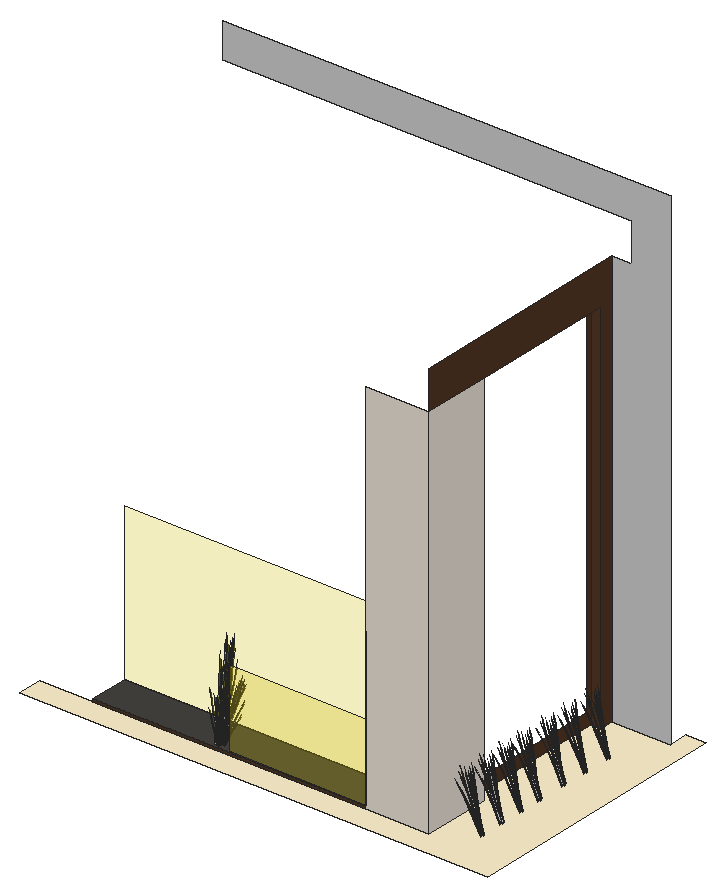
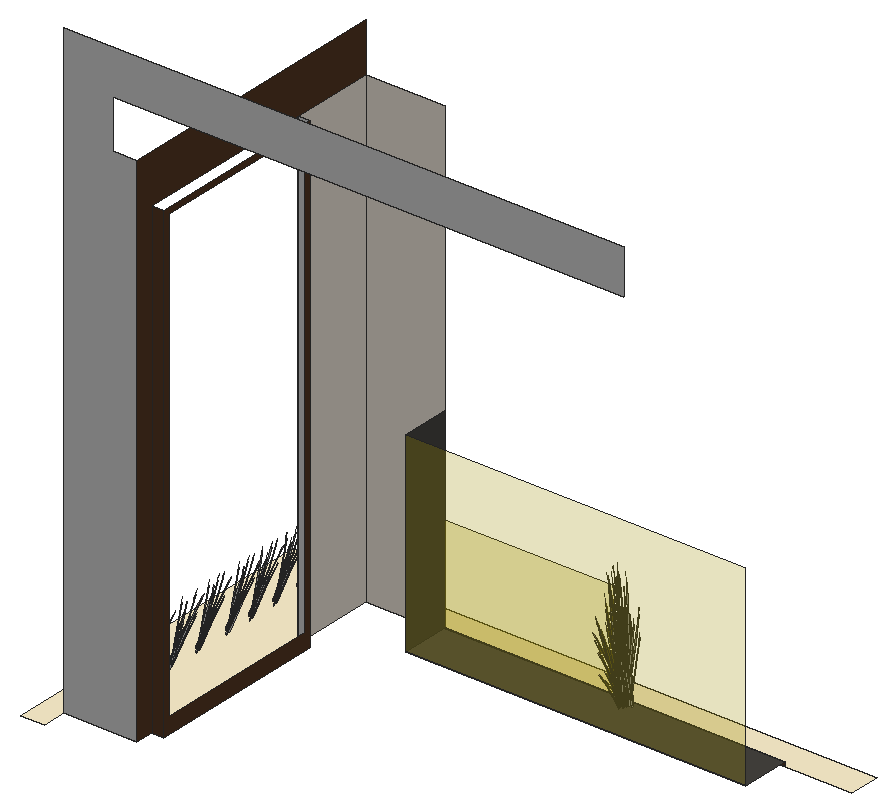
# SketchUp Ruby script. Lengths in inches.
U = 1.inch
M = Sketchup.active_model
def pt(a) = Geom::Point3d.new(a.map { |v| v * U })
def face(e, loops, mat)
  f = e.add_face(loops[0].map { |a| pt(a) })
  loops[1..].each { |l| e.add_face(l.map { |a| pt(a) }).erase! }
  f.material = f.back_material = mat if mat
  f
end
# faces: each face lists its corners as indices into pts; further lists are holes
def faces(e, pts, list, mat = nil) = list.each { |f| face(e, (f[0].is_a?(Array) ? f : [f]).map { |l| l.map { |i| pts[i] } }, mat) }
# xy, xz, yz: faces in a plane at the given z, y or x. An outline is a flat list of corners, or four numbers for a rectangle; further outlines are holes
def ring(l) = l.size == 4 ? [[l[0], l[1]], [l[2], l[1]], [l[2], l[3]], [l[0], l[3]]] : l.each_slice(2).to_a
def flat(e, list, mat, &to3) = list.each { |f| face(e, (f[0].is_a?(Array) ? f : [f]).map { |l| ring(l).map { |u, v| to3.(u, v) } }, mat) }
def xy(e, z, list, mat = nil) = flat(e, list, mat) { |x, y| [x, y, z] }
def xz(e, y, list, mat = nil) = flat(e, list, mat) { |x, z| [x, y, z] }
def yz(e, x, list, mat = nil) = flat(e, list, mat) { |y, z| [x, y, z] }
def lines(e, pts, list) = list.each { |a, b| e.add_line(pt(pts[a]), pt(pts[b])) }
# prism: a flat outline (further loops are holes) pulled along v
def prism(e, loops, v, mat = nil)
  f = face(e, loops, mat); d = Geom::Vector3d.new(v.map { |x| x * U })
  f.pushpull(f.normal.samedirection?(d) ? d.length : -d.length)
end
def box(e, o, s, mat = nil) = prism(e, [[o, [o[0] + s[0], o[1], o[2]], [o[0] + s[0], o[1] + s[1], o[2]], [o[0], o[1] + s[1], o[2]]]], [0, 0, s[2]], mat)
def at(x, y, z, deg = 0) = Geom::Transformation.translation(pt([x, y, z])) * Geom::Transformation.rotation(ORIGIN, Z_AXIS, deg.degrees)
def axes(o, x, y, z) = Geom::Transformation.new([*x, 0, *y, 0, *z, 0, *pt(o).to_a, 1])
def part(name) = M.definitions.add(name)
# library, detail: a bought-in or finely detailed component or shape, given as its bounding box
def library(name, o, s) = part(name).tap { |d| box(d.entities, o, s) }
def detail(e, o, s) = box(e.add_group.entities, o, s)
def put(e, d, t, mat = nil) = e.add_instance(d, t).tap { |i| i.material = mat if mat }
def group(e, t, mat = nil) = e.add_group.tap { |g| g.transformation = t; g.material = mat if mat }.entities
root = M.entities
M.materials.add("D01_Frost_White").color = [255, 242, 206]
M.materials.add("Glass_Basic_01").color = [255, 228, 0]
M.materials["Glass_Basic_01"].alpha = 0.25
M.materials.add("LightPink_Translucent").color = [144, 107, 117]
M.materials["LightPink_Translucent"].alpha = 0.75
M.materials.add("Marble_01_1K").color = [230, 221, 211]
M.materials.add("Wood_Planks_01_1K").color = [69, 67, 63]
M.materials.add("Wood_Veneer_15_1K").color = [81, 54, 35]
M.materials.add("[_0053_Ivory_]").color = [200, 200, 200]
c1 = part("blade")
p = [[2.15,0.21,22],[0,0.17,0],[0.09,0.45,0],[2.18,0.31,22],[2.29,0.31,22],[0.38,0.45,0],
  [2.48,0.24,33],[2.49,0.24,33],[2.48,0.22,33]]
faces(c1.entities,p,[[0,1,2,3],[4,5,2,3],[6,3,4,7],[8,0,3,6]])
c2 = part("seeds")
p = [[0.3,-0.1,1.38],[-0.01,-0.03,1.59],[-0.01,-0.03,0.03],[0.14,-0.07,-0.07],[0.29,-0.03,3],[0.15,0.01,3.11]]
faces(c2.entities,p,[[0,1,2,3],[1,0,4,5]],"LightPink_Translucent")
c3 = part("blade with seeds")
put(c3.entities,c1,at(0,0,0))
put(c3.entities,c2,axes([2.4,0.25,30.99],[1.5799,-0.05474,1.17369],[-0.12525,1.92788,0.29478],[-0.07173,-0.02425,1.56792]))
xy(root,127,[[377.51,83.15,665.51,83.15,665.51,251.15,653.51,251.15,653.51,239.15,617.51,239.15,617.51,230.15,611.51,230.15,611.51,140.15,617.51,140.15,617.51,98.15,377.51,98.15]],"D01_Frost_White")
xy(root,129,[[410.51,98.15,578.51,122.15]],"Wood_Planks_01_1K")
xz(root,98.15,[[494.51,129,578.51,177]],"Glass_Basic_01")
xz(root,98.15,[[578.51,127,617.51,360]],"Marble_01_1K")
xz(root,98.15,[[410.51,127,578.51,129]],"Wood_Veneer_15_1K")
xz(root,122.15,[[410.51,129,578.51,225]],"Glass_Basic_01")
xz(root,140.15,[[611.51,127,617.51,360]],"[_0053_Ivory_]")
xz(root,230.15,[[611.51,127,617.51,360]],"Wood_Veneer_15_1K")
xz(root,239.15,[[617.51,127,653.51,127,653.51,430,377.51,430,377.51,408,629.51,408,629.51,384,617.51,384]],"[_0053_Ivory_]")
yz(root,578.51,[[98.15,129,122.15,225]],"Wood_Planks_01_1K")
yz(root,611.51,[[[140.15,127,230.15,360],[143.15,135,227.15,357]]],"Wood_Veneer_15_1K")
yz(root,617.51,[[98.15,127,140.15,360]],"Marble_01_1K")
yz(root,617.51,[[230.15,127,239.15,127,239.15,384,98.15,384,98.15,360,230.15,360]],"Wood_Veneer_15_1K")
put(root,c3,axes([484.17,100.16,128.68],[0.56663,0.1556,-0.30978],[-0.14267,0.54795,0.30978],[0.11423,-0.06319,1.38974]),"[_0053_Ivory_]")
put(root,c3,axes([485.75,99.5,129.24],[-0.17264,0.12729,1.43002],[-0.51703,-0.22279,-0.30754],[0.09584,-0.27707,0.61141]),"[_0053_Ivory_]")
put(root,c3,axes([487.11,102.46,129.13],[0,-0.62885,0.49651],[0.67951,0,0],[0,0.14322,1.57504]),"[_0053_Ivory_]")
put(root,c3,axes([487.4,103.04,128.67],[0,0.62885,-0.49651],[-0.67951,0,0],[0,0.14322,1.57504]),"[_0053_Ivory_]")
put(root,c3,axes([484.04,99.91,128.67],[0.56842,-0.31443,-0.49651],[0.33976,0.56381,0],[0.12946,-0.07161,1.57504]),"[_0053_Ivory_]")
put(root,c3,axes([484.77,103.74,130.53],[-0.13883,-0.2019,1.71376],[0.64153,-0.16998,0.13857],[0.14499,0.31697,0.73262]),"[_0053_Ivory_]")
put(root,c3,axes([485.18,101.47,129.27],[0.11717,-0.56122,0.1448],[0.57245,0.09742,-0.41347],[0.10418,0.05763,1.26744]),"[_0053_Ivory_]")
put(root,c3,axes([485.99,100.5,129.13],[-0.56842,-0.31443,0.49651],[0.33976,-0.56381,0],[0.12946,0.07161,1.57504]),"[_0053_Ivory_]")
put(root,c3,axes([486.17,100.44,131.63],[0.0158,-0.58168,-0.71045],[0.66548,0.03907,0.08574],[0.07023,-0.24643,1.00501]),"[_0053_Ivory_]")
put(root,c3,axes([485.5,103.78,128.84],[0.63764,-0.21337,-0.19198],[0.22406,0.61462,0.00008],[0.07038,-0.02358,1.73897]),"[_0053_Ivory_]")
put(root,c3,axes([485.51,101.95,128.86],[0.36485,0.52782,-0.44739],[-0.55265,0.37168,0.21531],[0.11807,0.06531,1.43643]),"[_0053_Ivory_]")
put(root,c3,axes([486.44,100.09,131.18],[0.41095,-0.33109,-0.35414],[0.38901,0.37805,0.4572],[0.05919,-0.19208,0.87481]),"[_0053_Ivory_]")
put(root,c3,axes([486.54,104.35,129.42],[-0.34197,-0.18082,1.1486],[0.44156,-0.18372,0.84392],[0.1191,0.15563,0.25299]),"[_0053_Ivory_]")
put(root,c3,axes([485.32,104.15,129.24],[0.01072,-0.20846,1.43002],[0.51218,-0.23285,-0.30754],[0.15811,0.2495,0.61141]),"[_0053_Ivory_]")
put(root,c3,axes([484.71,101.2,128.71],[0.40909,-0.47266,-0.62353],[0.50819,0.4286,-0.16365],[0.16393,-0.11791,1.37633]),"[_0053_Ivory_]")
put(root,c3,axes([486.51,100.78,128.68],[0.14267,0.54795,-0.30978],[-0.56663,0.1556,0.30978],[0.11423,0.06319,1.38974]),"[_0053_Ivory_]")
put(root,c3,axes([487.57,102.57,129.03],[0.75945,0,0],[0,0.70283,-0.51607],[0,0.16007,1.63711]),"[_0053_Ivory_]")
put(root,c3,axes([485.12,101.66,129.32],[0.61322,-0.4175,-0.29095],[0.40778,0.58992,-0.50002],[0.1513,0.05991,1.59708]),"[_0053_Ivory_]")
put(root,c3,axes([486.59,105.17,129.32],[-0.38947,-0.01972,1.0506],[0.25721,-0.41888,0.58006],[0.15386,0.14882,0.8241]),"[_0053_Ivory_]")
put(root,c3,axes([485.42,100.15,130.53],[-0.11309,0.21615,1.71376],[-0.47441,-0.44731,0.13857],[0.21402,-0.27879,0.73262]),"[_0053_Ivory_]")
put(root,c3,axes([483.57,101.28,128.25],[-0.59782,0.25177,1.28929],[-0.19028,-0.72239,0.50096],[0.36709,0.01202,1.46642]),"[_0053_Ivory_]")
put(root,c3,axes([485.77,104.6,131.33],[0.59932,-0.14948,-0.51099],[0.10484,0.56611,-0.3958],[0.16097,0.16223,0.97773]),"[_0053_Ivory_]")
put(root,c3,axes([486.32,100.17,129.03],[0.37973,-0.63014,0],[0.6353,0.35142,-0.51607],[0.14469,0.08004,1.63711]),"[_0053_Ivory_]")
put(root,c3,axes([486.95,99.89,128.15],[-0.0909,-0.04954,1.76342],[-0.2335,-0.55347,-0.26939],[0.15752,-0.1502,0.30037]),"[_0053_Ivory_]")
put(root,c3,axes([486.66,100.55,128.67],[0.56842,0.31443,-0.49651],[-0.33976,0.56381,0],[0.12946,0.07161,1.57504]),"[_0053_Ivory_]")
put(root,c3,axes([486.64,105.02,128.15],[0.04425,-0.09079,1.76342],[0.55709,-0.26738,-0.26939],[0.16889,0.13839,0.30037]),"[_0053_Ivory_]")
put(root,c3,axes([486.94,101.22,131.33],[-0.15602,-0.5742,-0.51099],[0.59087,-0.10045,-0.3958],[0.16933,-0.15423,0.97773]),"[_0053_Ivory_]")
put(root,c3,axes([487.97,104.18,130.58],[-0.11624,-0.52862,-0.03492],[0.54943,-0.12153,-0.15832],[0.11473,0.03351,0.52218]),"[_0053_Ivory_]")
put(root,c3,axes([485.84,101.75,128.71],[0.63179,0.1031,-0.62353],[-0.13332,0.63596,-0.16365],[0.18854,0.07706,1.37633]),"[_0053_Ivory_]")
put(root,c3,axes([488.53,102.125,128.91],[-0.37654,-0.40212,-0.06488],[0.4124,-0.36845,-0.29416],[0.11685,-0.02594,0.97024]),"[_0053_Ivory_]")
put(root,c3,axes([487.66,100.08,129.42],[-0.2023,0.32011,1.1486],[-0.17388,-0.43009,0.84392],[0.16708,-0.10777,0.25299]),"[_0053_Ivory_]")
put(root,c3,axes([485.7,103.11,130.53],[-0.2256,-0.10835,1.71376],[0.46687,-0.45453,0.13857],[0.29098,0.20505,0.73262]),"[_0053_Ivory_]")
put(root,c3,axes([487.37,101.28,131.18],[0.52868,-0.08987,-0.35414],[0.1396,0.51376,0.4572],[0.1515,-0.13799,0.87481]),"[_0053_Ivory_]")
put(root,c3,axes([486.95,101.45,131.63],[0.31725,-0.49618,-0.71045],[0.55593,0.35263,0.08574],[0.18942,-0.17977,1.00501]),"[_0053_Ivory_]")
put(root,c3,axes([486.95,104.12,131.18],[0.34557,0.39372,-0.35414],[-0.39459,0.37271,0.4572],[0.20048,0.05671,0.87481]),"[_0053_Ivory_]")
put(root,c3,axes([487.21,102.5,131.33],[0.16454,-0.57202,-0.51099],[0.56413,0.19607,-0.3958],[0.22713,-0.05245,0.97773]),"[_0053_Ivory_]")
put(root,c3,axes([488.625,102.86,129.42],[-0.37526,0.10382,1.1486],[0.17664,-0.42906,0.84392],[0.19907,0.02936,0.25299]),"[_0053_Ivory_]")
put(root,c3,axes([487.41,101,129.24],[-0.21697,-0.01863,1.43002],[-0.22228,-0.49966,-0.30754],[0.26655,-0.14135,0.61141]),"[_0053_Ivory_]")
put(root,c3,axes([487.56,102.76,131.18],[0.50475,0.17543,-0.35414],[-0.14722,0.5118,0.4572],[0.20322,-0.04693,0.87481]),"[_0053_Ivory_]")
put(root,c3,axes([486.58,103.86,131.63],[0.60713,0.01514,-0.71045],[-0.04078,0.63759,0.08574],[0.25721,0.06729,1.00501]),"[_0053_Ivory_]")
put(root,c3,axes([487.8125,102.66,128.64],[-0.39118,0.07547,1.41583],[-0.06226,-0.6007,0.08104],[0.27398,-0.09092,0.80566]),"[_0053_Ivory_]")
put(root,c3,axes([488.24,102.26,128.15],[-0.03174,-0.09547,1.76342],[0.22015,-0.55846,-0.26939],[0.22208,-0.00803,0.30037]),"[_0053_Ivory_]")
put(root,c3,axes([486.18,102.12,130.53],[-0.25192,0.01424,1.71376],[0.16712,-0.61729,0.13857],[0.35901,0.03818,0.73262]),"[_0053_Ivory_]")
put(root,c3,axes([487.1,102.7,131.63],[0.53369,-0.27773,-0.71045],[0.29743,0.5717,0.08574],[0.25786,-0.06494,1.00501]),"[_0053_Ivory_]")
put(root,c3,axes([487.92,103.55,129.24],[-0.14627,-0.15466,1.43002],[0.19032,-0.51164,-0.30754],[0.29594,0.06931,0.61141]),"[_0053_Ivory_]")
put(root,c3,axes([641.08,108.52,130.53],[0.25192,-0.01424,1.71376],[-0.16712,0.61729,0.13857],[-0.35901,-0.03818,0.73262]),"[_0053_Ivory_]")
put(root,c3,axes([641.08,123.58,130.53],[0.25192,-0.01424,1.71376],[-0.16712,0.61729,0.13857],[-0.35901,-0.03818,0.73262]),"[_0053_Ivory_]")
put(root,c3,axes([641.08,138.5,130.53],[0.25192,-0.01424,1.71376],[-0.16712,0.61729,0.13857],[-0.35901,-0.03818,0.73262]),"[_0053_Ivory_]")
put(root,c3,axes([641.08,152.78,130.53],[0.25192,-0.01424,1.71376],[-0.16712,0.61729,0.13857],[-0.35901,-0.03818,0.73262]),"[_0053_Ivory_]")
put(root,c3,axes([641.08,171.26,130.53],[0.25192,-0.01424,1.71376],[-0.16712,0.61729,0.13857],[-0.35901,-0.03818,0.73262]),"[_0053_Ivory_]")
put(root,c3,axes([641.08,188.02,130.53],[0.25192,-0.01424,1.71376],[-0.16712,0.61729,0.13857],[-0.35901,-0.03818,0.73262]),"[_0053_Ivory_]")
put(root,c3,axes([641.08,205.61,130.53],[0.25192,-0.01424,1.71376],[-0.16712,0.61729,0.13857],[-0.35901,-0.03818,0.73262]),"[_0053_Ivory_]")
put(root,c3,axes([641.1875,109.61,130.53],[0.21074,-0.13302,1.71376],[0.17741,0.61464,0.13857],[-0.33083,0.13891,0.73262]),"[_0053_Ivory_]")
put(root,c3,axes([641.1875,124.67,130.53],[0.21074,-0.13302,1.71376],[0.17741,0.61464,0.13857],[-0.33083,0.13891,0.73262]),"[_0053_Ivory_]")
put(root,c3,axes([641.1875,139.59,130.53],[0.21074,-0.13302,1.71376],[0.17741,0.61464,0.13857],[-0.33083,0.13891,0.73262]),"[_0053_Ivory_]")
put(root,c3,axes([641.1875,153.86,130.53],[0.21074,-0.13302,1.71376],[0.17741,0.61464,0.13857],[-0.33083,0.13891,0.73262]),"[_0053_Ivory_]")
put(root,c3,axes([641.1875,172.35,130.53],[0.21074,-0.13302,1.71376],[0.17741,0.61464,0.13857],[-0.33083,0.13891,0.73262]),"[_0053_Ivory_]")
put(root,c3,axes([641.1875,189.11,130.53],[0.21074,-0.13302,1.71376],[0.17741,0.61464,0.13857],[-0.33083,0.13891,0.73262]),"[_0053_Ivory_]")
put(root,c3,axes([641.1875,206.7,130.53],[0.21074,-0.13302,1.71376],[0.17741,0.61464,0.13857],[-0.33083,0.13891,0.73262]),"[_0053_Ivory_]")
put(root,c3,axes([640.53,110.65,129.24],[0.21107,0.05162,1.43002],[0.13604,0.52729,-0.30754],[-0.28671,0.0987,0.61141]),"[_0053_Ivory_]")
put(root,c3,axes([640.53,125.72,129.24],[0.21107,0.05162,1.43002],[0.13604,0.52729,-0.30754],[-0.28671,0.0987,0.61141]),"[_0053_Ivory_]")
put(root,c3,axes([640.53,140.63,129.24],[0.21107,0.05162,1.43002],[0.13604,0.52729,-0.30754],[-0.28671,0.0987,0.61141]),"[_0053_Ivory_]")
put(root,c3,axes([640.53,154.91,129.24],[0.21107,0.05162,1.43002],[0.13604,0.52729,-0.30754],[-0.28671,0.0987,0.61141]),"[_0053_Ivory_]")
put(root,c3,axes([640.53,173.39,129.24],[0.21107,0.05162,1.43002],[0.13604,0.52729,-0.30754],[-0.28671,0.0987,0.61141]),"[_0053_Ivory_]")
put(root,c3,axes([640.53,190.15,129.24],[0.21107,0.05162,1.43002],[0.13604,0.52729,-0.30754],[-0.28671,0.0987,0.61141]),"[_0053_Ivory_]")
put(root,c3,axes([640.53,207.74,129.24],[0.21107,0.05162,1.43002],[0.13604,0.52729,-0.30754],[-0.28671,0.0987,0.61141]),"[_0053_Ivory_]")
put(root,c3,axes([642.4,108.97,130],[0.17264,-0.09097,1.77064],[0.05953,0.63516,0.13857],[-0.37394,0.08428,0.63284]),"[_0053_Ivory_]")
put(root,c3,axes([642.4,124.03,130],[0.17264,-0.09097,1.77064],[0.05953,0.63516,0.13857],[-0.37394,0.08428,0.63284]),"[_0053_Ivory_]")
put(root,c3,axes([642.4,138.95,130],[0.17264,-0.09097,1.77064],[0.05953,0.63516,0.13857],[-0.37394,0.08428,0.63284]),"[_0053_Ivory_]")
put(root,c3,axes([642.4,153.22,130],[0.17264,-0.09097,1.77064],[0.05953,0.63516,0.13857],[-0.37394,0.08428,0.63284]),"[_0053_Ivory_]")
put(root,c3,axes([642.4,171.7,130],[0.17264,-0.09097,1.77064],[0.05953,0.63516,0.13857],[-0.37394,0.08428,0.63284]),"[_0053_Ivory_]")
put(root,c3,axes([642.4,188.46,130],[0.17264,-0.09097,1.77064],[0.05953,0.63516,0.13857],[-0.37394,0.08428,0.63284]),"[_0053_Ivory_]")
put(root,c3,axes([642.4,206.06,130],[0.17264,-0.09097,1.77064],[0.05953,0.63516,0.13857],[-0.37394,0.08428,0.63284]),"[_0053_Ivory_]")
put(root,c3,axes([641.83,107.95,131.63],[-0.60713,-0.01514,-0.71045],[0.04078,-0.63759,0.08574],[-0.25721,-0.06729,1.00501]),"[_0053_Ivory_]")
put(root,c3,axes([641.83,123.01,131.63],[-0.60713,-0.01514,-0.71045],[0.04078,-0.63759,0.08574],[-0.25721,-0.06729,1.00501]),"[_0053_Ivory_]")
put(root,c3,axes([641.83,137.93,131.63],[-0.60713,-0.01514,-0.71045],[0.04078,-0.63759,0.08574],[-0.25721,-0.06729,1.00501]),"[_0053_Ivory_]")
put(root,c3,axes([641.83,152.2,131.63],[-0.60713,-0.01514,-0.71045],[0.04078,-0.63759,0.08574],[-0.25721,-0.06729,1.00501]),"[_0053_Ivory_]")
put(root,c3,axes([641.83,170.6875,131.63],[-0.60713,-0.01514,-0.71045],[0.04078,-0.63759,0.08574],[-0.25721,-0.06729,1.00501]),"[_0053_Ivory_]")
put(root,c3,axes([641.83,187.45,131.63],[-0.60713,-0.01514,-0.71045],[0.04078,-0.63759,0.08574],[-0.25721,-0.06729,1.00501]),"[_0053_Ivory_]")
put(root,c3,axes([641.83,205.04,131.63],[-0.60713,-0.01514,-0.71045],[0.04078,-0.63759,0.08574],[-0.25721,-0.06729,1.00501]),"[_0053_Ivory_]")
put(root,c3,axes([641.35,108.1,129.24],[0.11858,0.17508,1.43002],[-0.27325,0.4759,-0.30754],[-0.28057,-0.11375,0.61141]),"[_0053_Ivory_]")
put(root,c3,axes([641.35,123.17,129.24],[0.11858,0.17508,1.43002],[-0.27325,0.4759,-0.30754],[-0.28057,-0.11375,0.61141]),"[_0053_Ivory_]")
put(root,c3,axes([641.35,138.08,129.24],[0.11858,0.17508,1.43002],[-0.27325,0.4759,-0.30754],[-0.28057,-0.11375,0.61141]),"[_0053_Ivory_]")
put(root,c3,axes([641.35,152.36,129.24],[0.11858,0.17508,1.43002],[-0.27325,0.4759,-0.30754],[-0.28057,-0.11375,0.61141]),"[_0053_Ivory_]")
put(root,c3,axes([641.35,170.84,129.24],[0.11858,0.17508,1.43002],[-0.27325,0.4759,-0.30754],[-0.28057,-0.11375,0.61141]),"[_0053_Ivory_]")
put(root,c3,axes([641.35,187.6,129.24],[0.11858,0.17508,1.43002],[-0.27325,0.4759,-0.30754],[-0.28057,-0.11375,0.61141]),"[_0053_Ivory_]")
put(root,c3,axes([641.35,205.19,129.24],[0.11858,0.17508,1.43002],[-0.27325,0.4759,-0.30754],[-0.28057,-0.11375,0.61141]),"[_0053_Ivory_]")
put(root,c3,axes([640.86,109.05,131.18],[-0.50475,-0.17543,-0.35414],[0.14722,-0.5118,0.4572],[-0.20322,0.04693,0.87481]),"[_0053_Ivory_]")
put(root,c3,axes([640.86,124.11,131.18],[-0.50475,-0.17543,-0.35414],[0.14722,-0.5118,0.4572],[-0.20322,0.04693,0.87481]),"[_0053_Ivory_]")
put(root,c3,axes([640.86,139.03,131.18],[-0.50475,-0.17543,-0.35414],[0.14722,-0.5118,0.4572],[-0.20322,0.04693,0.87481]),"[_0053_Ivory_]")
put(root,c3,axes([640.86,153.31,131.18],[-0.50475,-0.17543,-0.35414],[0.14722,-0.5118,0.4572],[-0.20322,0.04693,0.87481]),"[_0053_Ivory_]")
put(root,c3,axes([640.86,171.79,131.18],[-0.50475,-0.17543,-0.35414],[0.14722,-0.5118,0.4572],[-0.20322,0.04693,0.87481]),"[_0053_Ivory_]")
put(root,c3,axes([640.86,188.55,131.18],[-0.50475,-0.17543,-0.35414],[0.14722,-0.5118,0.4572],[-0.20322,0.04693,0.87481]),"[_0053_Ivory_]")
put(root,c3,axes([640.86,206.14,131.18],[-0.50475,-0.17543,-0.35414],[0.14722,-0.5118,0.4572],[-0.20322,0.04693,0.87481]),"[_0053_Ivory_]")
put(root,c3,axes([641.56,107.53,130.53],[0.2256,0.10835,1.71376],[-0.46687,0.45453,0.13857],[-0.29098,-0.20505,0.73262]),"[_0053_Ivory_]")
put(root,c3,axes([641.56,122.59,130.53],[0.2256,0.10835,1.71376],[-0.46687,0.45453,0.13857],[-0.29098,-0.20505,0.73262]),"[_0053_Ivory_]")
put(root,c3,axes([641.56,137.51,130.53],[0.2256,0.10835,1.71376],[-0.46687,0.45453,0.13857],[-0.29098,-0.20505,0.73262]),"[_0053_Ivory_]")
put(root,c3,axes([641.56,151.79,130.53],[0.2256,0.10835,1.71376],[-0.46687,0.45453,0.13857],[-0.29098,-0.20505,0.73262]),"[_0053_Ivory_]")
put(root,c3,axes([641.56,170.27,130.53],[0.2256,0.10835,1.71376],[-0.46687,0.45453,0.13857],[-0.29098,-0.20505,0.73262]),"[_0053_Ivory_]")
put(root,c3,axes([641.56,187.03,130.53],[0.2256,0.10835,1.71376],[-0.46687,0.45453,0.13857],[-0.29098,-0.20505,0.73262]),"[_0053_Ivory_]")
put(root,c3,axes([641.56,204.62,130.53],[0.2256,0.10835,1.71376],[-0.46687,0.45453,0.13857],[-0.29098,-0.20505,0.73262]),"[_0053_Ivory_]")
put(root,c3,axes([641.21,109.3125,131.33],[-0.16454,0.57202,-0.51099],[-0.56413,-0.19607,-0.3958],[-0.22713,0.05245,0.97773]),"[_0053_Ivory_]")
put(root,c3,axes([641.21,124.375,131.33],[-0.16454,0.57202,-0.51099],[-0.56413,-0.19607,-0.3958],[-0.22713,0.05245,0.97773]),"[_0053_Ivory_]")
put(root,c3,axes([641.21,139.29,131.33],[-0.16454,0.57202,-0.51099],[-0.56413,-0.19607,-0.3958],[-0.22713,0.05245,0.97773]),"[_0053_Ivory_]")
put(root,c3,axes([641.21,153.57,131.33],[-0.16454,0.57202,-0.51099],[-0.56413,-0.19607,-0.3958],[-0.22713,0.05245,0.97773]),"[_0053_Ivory_]")
put(root,c3,axes([641.21,172.05,131.33],[-0.16454,0.57202,-0.51099],[-0.56413,-0.19607,-0.3958],[-0.22713,0.05245,0.97773]),"[_0053_Ivory_]")
put(root,c3,axes([641.21,188.8125,131.33],[-0.16454,0.57202,-0.51099],[-0.56413,-0.19607,-0.3958],[-0.22713,0.05245,0.97773]),"[_0053_Ivory_]")
put(root,c3,axes([641.21,206.4,131.33],[-0.16454,0.57202,-0.51099],[-0.56413,-0.19607,-0.3958],[-0.22713,0.05245,0.97773]),"[_0053_Ivory_]")
put(root,c3,axes([641.63,108.08,131.33],[-0.44101,0.41656,-0.51099],[-0.38623,-0.44004,-0.3958],[-0.22407,-0.06338,0.97773]),"[_0053_Ivory_]")
put(root,c3,axes([641.63,123.14,131.33],[-0.44101,0.41656,-0.51099],[-0.38623,-0.44004,-0.3958],[-0.22407,-0.06338,0.97773]),"[_0053_Ivory_]")
put(root,c3,axes([641.63,138.06,131.33],[-0.44101,0.41656,-0.51099],[-0.38623,-0.44004,-0.3958],[-0.22407,-0.06338,0.97773]),"[_0053_Ivory_]")
put(root,c3,axes([641.63,152.33,131.33],[-0.44101,0.41656,-0.51099],[-0.38623,-0.44004,-0.3958],[-0.22407,-0.06338,0.97773]),"[_0053_Ivory_]")
put(root,c3,axes([641.63,170.82,131.33],[-0.44101,0.41656,-0.51099],[-0.38623,-0.44004,-0.3958],[-0.22407,-0.06338,0.97773]),"[_0053_Ivory_]")
